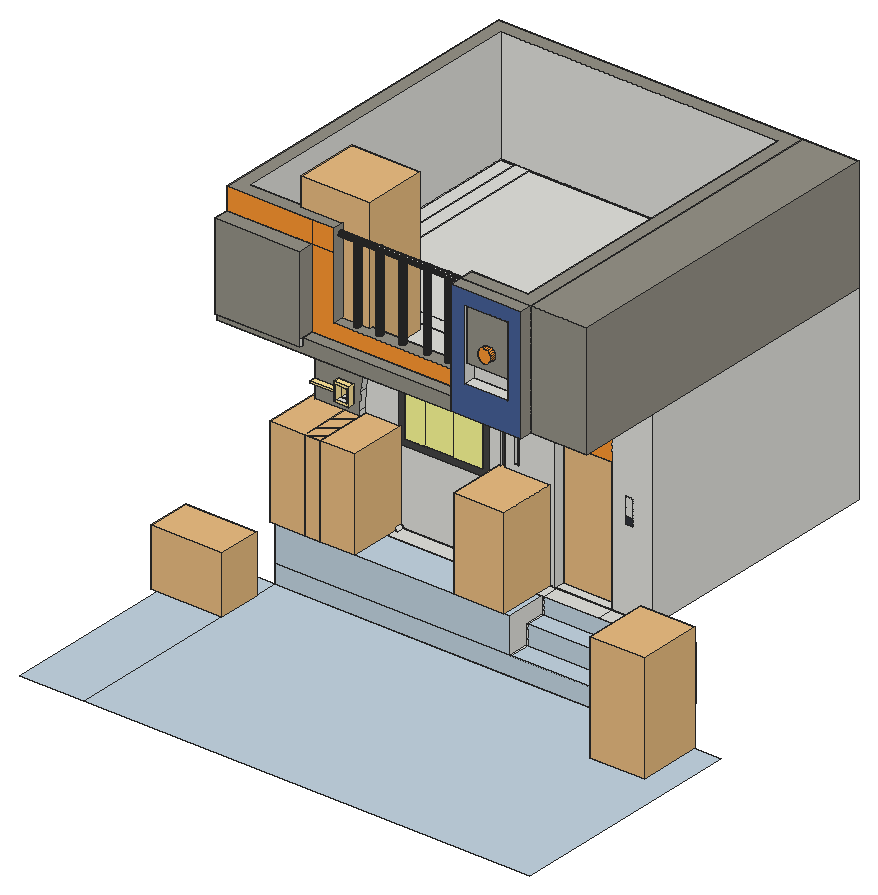
# SketchUp Ruby script. Lengths in inches.
U = 1.inch
M = Sketchup.active_model
def pt(a) = Geom::Point3d.new(a.map { |v| v * U })
def face(e, loops, mat)
  f = e.add_face(loops[0].map { |a| pt(a) })
  loops[1..].each { |l| e.add_face(l.map { |a| pt(a) }).erase! }
  f.material = f.back_material = mat if mat
  f
end
# faces: each face lists its corners as indices into pts; further lists are holes
def faces(e, pts, list, mat = nil) = list.each { |f| face(e, (f[0].is_a?(Array) ? f : [f]).map { |l| l.map { |i| pts[i] } }, mat) }
# xy, xz, yz: faces in a plane at the given z, y or x. An outline is a flat list of corners, or four numbers for a rectangle; further outlines are holes
def ring(l) = l.size == 4 ? [[l[0], l[1]], [l[2], l[1]], [l[2], l[3]], [l[0], l[3]]] : l.each_slice(2).to_a
def flat(e, list, mat, &to3) = list.each { |f| face(e, (f[0].is_a?(Array) ? f : [f]).map { |l| ring(l).map { |u, v| to3.(u, v) } }, mat) }
def xy(e, z, list, mat = nil) = flat(e, list, mat) { |x, y| [x, y, z] }
def xz(e, y, list, mat = nil) = flat(e, list, mat) { |x, z| [x, y, z] }
def yz(e, x, list, mat = nil) = flat(e, list, mat) { |y, z| [x, y, z] }
def lines(e, pts, list) = list.each { |a, b| e.add_line(pt(pts[a]), pt(pts[b])) }
# prism: a flat outline (further loops are holes) pulled along v
def prism(e, loops, v, mat = nil)
  f = face(e, loops, mat); d = Geom::Vector3d.new(v.map { |x| x * U })
  f.pushpull(f.normal.samedirection?(d) ? d.length : -d.length)
end
def box(e, o, s, mat = nil) = prism(e, [[o, [o[0] + s[0], o[1], o[2]], [o[0] + s[0], o[1] + s[1], o[2]], [o[0], o[1] + s[1], o[2]]]], [0, 0, s[2]], mat)
def at(x, y, z, deg = 0) = Geom::Transformation.translation(pt([x, y, z])) * Geom::Transformation.rotation(ORIGIN, Z_AXIS, deg.degrees)
def axes(o, x, y, z) = Geom::Transformation.new([*x, 0, *y, 0, *z, 0, *pt(o).to_a, 1])
def part(name) = M.definitions.add(name)
# library, detail: a bought-in or finely detailed component or shape, given as its bounding box
def library(name, o, s) = part(name).tap { |d| box(d.entities, o, s) }
def detail(e, o, s) = box(e.add_group.entities, o, s)
def put(e, d, t, mat = nil) = e.add_instance(d, t).tap { |i| i.material = mat if mat }
def group(e, t, mat = nil) = e.add_group.tap { |g| g.transformation = t; g.material = mat if mat }.entities
root = M.entities
M.materials.add("[Color C04]").color = [255, 153, 50]
M.materials.add("[Color D02]").color = [255, 229, 153]
M.materials.add("[Color E02]").color = [255, 255, 153]
M.materials.add("[Formica Blue]").color = [71, 97, 152]
M.materials.add("[Formica Graystone]").color = [149, 146, 135]
M.materials.add("[Formica Laminate Dark]").color = [50, 53, 60]
M.materials.add("[Granite Dark Gray]").color = [69, 68, 68]
M.materials.add("[Terrazzo Light Blue]").color = [196, 214, 227]
c1 = library("Decorative Plant",[-0.35,-0.24,0],[4.14,4.48,6.875])
c2 = library("blómastandur (1)",[6.48,-34.53,1.97],[34.7,40.11,68.37])
c3 = library("plantas+internas",[0,0,0],[44.91,27.47,36.11])
c4 = library("Door",[183.55,487.57,0],[5.16,42.5,84])
xy(root,-34.375,[[40.65,150.875,189.96,186.6875],[189.96,150.875,277.77,186.6875]])
xy(root,-34.375,[[0,0,40.65,150.875],[40.65,0,322.27,150.875]],"[Terrazzo Light Blue]")
xy(root,-22.29,[[40.65,150.875,189.02,163.875],[189.02,150.875,189.96,163.875]])
xy(root,-22.29,[[189.96,150.875,277.77,163.875]],"[Terrazzo Light Blue]")
xy(root,-10.2,[[40.65,163.875,189.02,176.1875],[189.02,163.875,189.96,176.1875]])
xy(root,-10.2,[[189.96,163.875,277.77,176.1875]],"[Terrazzo Light Blue]")
xy(root,0,[[40.65,176.1875,189.96,176.1875,189.96,186.6875,93.13,186.6875,93.13,182.375,40.65,182.375],[189.96,176.1875,225.02,186.6875],[225.02,176.1875,250.96,186.6875],[250.96,176.1875,277.77,186.6875],[40.65,182.375,93.13,186.6875],
  [40.65,186.6875,40.65,349.1875,250.96,349.1875,250.96,186.6875,225.02,186.6875,225.02,195.6875,241.96,195.6875,241.96,340.1875,49.65,340.1875,49.65,195.6875,189.02,195.6875,189.02,186.6875],[189.02,186.6875,225.02,195.6875],[49.65,195.6875,241.96,340.1875]])
xy(root,0,[[40.65,150.5625,189.02,176.1875]],"[Terrazzo Light Blue]")
xy(root,29.77,[[55.61,182.375,65.29,186.6875]])
xy(root,29.77,[[55.61,178.4375,65.29,182.375]],"[Color D02]")
xy(root,31.08,[[56.93,178.4375,63.97,182.375],[56.93,182.375,63.97,186.6875]],"[Color D02]")
xy(root,34.99,[[40.65,182.375,55.61,186.6875]])
xy(root,34.99,[[40.65,178.4375,55.61,182.375]],"[Color D02]")
xy(root,36.67,[[40.65,182.375,55.61,186.6875]])
xy(root,36.67,[[40.65,178.4375,55.61,182.375]],"[Color D02]")
xy(root,39.6875,[[154.5625,186.6875,157,188]])
xy(root,39.9375,[[56.93,178.4375,63.97,182.375],[56.93,182.375,63.97,186.6875]],"[Color D02]")
xy(root,41.25,[[55.61,182.375,65.29,186.6875]])
xy(root,41.25,[[55.61,178.4375,65.29,182.375]],"[Color D02]")
xy(root,51.2,[[93.97,186.6875,143.27,195.6875]])
xy(root,61.125,[[163.3,186.6875,166.05,188.1875]])
xy(root,62.33,[[55.61,182.375,65.29,186.6875]])
xy(root,62.33,[[55.61,178.4375,65.29,182.375]],"[Color D02]")
xy(root,63.64,[[56.93,178.4375,63.97,182.375],[56.93,182.375,63.97,186.6875]])
xy(root,67.54,[[40.65,182.375,55.61,186.6875],[40.65,186.6875,55.61,186.9375]])
xy(root,67.54,[[40.65,178.4375,55.61,182.375]],"[Color D02]")
xy(root,68.76,[[40.65,182.375,55.61,186.6875],[40.65,186.6875,55.61,186.9375]])
xy(root,68.76,[[40.65,178.4375,55.61,182.375]],"[Color D02]")
xy(root,72.5,[[56.93,178.4375,63.97,182.375],[56.93,182.375,63.97,186.6875]],"[Color D02]")
xy(root,73.8125,[[55.61,182.375,65.29,186.6875]])
xy(root,73.8125,[[55.61,178.4375,65.29,182.375]],"[Color D02]")
xy(root,84,[[189.02,186.6875,225.02,195.6875]])
xy(root,87.9375,[[171.8,186.6875,174.67,187.875]])
xy(root,89.08,[[55.61,182.375,65.29,186.6875]])
xy(root,89.08,[[55.61,178.4375,65.29,182.375]],"[Color D02]")
xy(root,90.39,[[56.93,178.4375,63.97,182.375],[56.93,182.375,63.97,186.6875]])
xy(root,93.49,[[93.97,186.6875,143.27,195.6875,143.27,186.6875],[93.97,186.6875,93.97,195.6875,143.27,195.6875]])
xy(root,94.2,[[40.65,182.375,55.61,185.875],[40.65,185.875,55.61,186.6875]])
xy(root,94.2,[[40.65,178.4375,55.61,182.375]],"[Color D02]")
xy(root,95.88,[[40.65,182.375,55.61,185.875],[40.65,185.875,55.61,186.6875]])
xy(root,95.88,[[40.65,178.4375,55.61,182.375]],"[Color D02]")
xy(root,99.25,[[56.93,178.4375,63.97,182.375],[56.93,182.375,63.97,186.6875]],"[Color D02]")
xy(root,100.5625,[[55.61,182.375,65.29,186.6875]])
xy(root,100.5625,[[55.61,178.4375,65.29,182.375]],"[Color D02]")
xy(root,120,[[40.65,182.375,93.13,186.6875],[[40.65,186.6875,154.5625,186.6875,154.5625,188,157,188,157,186.6875,163.3,186.6875,163.3,188.1875,166.05,188.1875,166.05,186.6875,171.8,186.6875,171.8,187.875,174.67,187.875,174.67,186.6875,250.96,186.6875,250.96,349.1875,40.65,349.1875],[49.65,195.6875,241.96,340.1875]]])
xz(root,150.875,[[40.65,-34.375,277.77,-22.29]],"[Terrazzo Light Blue]")
xz(root,163.875,[[40.65,-22.29,189.02,-10.2],[189.02,-22.29,189.96,-10.2]])
xz(root,163.875,[[189.96,-22.29,277.77,-10.2]],"[Terrazzo Light Blue]")
xz(root,176.1875,[[40.65,-10.2,189.02,0],[189.02,-10.2,189.96,0]])
xz(root,176.1875,[[189.96,-10.2,277.77,0]],"[Terrazzo Light Blue]")
xz(root,178.4375,[[[55.61,29.77,65.29,41.25],[56.93,31.08,63.97,39.9375]],[40.65,34.99,55.61,36.67],[[55.61,62.33,65.29,73.8125],[56.93,63.64,63.97,72.5]],[40.65,67.54,55.61,68.76],[[55.61,89.08,65.29,100.5625],[56.93,90.39,63.97,99.25]],
  [40.65,94.2,55.61,95.88]],"[Color D02]")
xz(root,182.375,[[[55.61,29.77,65.29,41.25],[56.93,31.08,63.97,39.9375]],[40.65,34.99,55.61,36.67],[[55.61,62.33,65.29,73.8125],[56.93,63.64,63.97,72.5]],[40.65,67.54,55.61,68.76],[[55.61,89.08,65.29,100.5625],[56.93,90.39,63.97,99.25]],
  [40.65,94.2,55.61,95.88]])
xz(root,182.375,[[40.65,0,93.13,0,85.93,8.4,79.86,17.65,75.04,27.61,71.53,38.1,69.41,48.96,68.7,60,69.41,71.04,71.53,81.9,75.04,92.39,79.86,102.35,85.93,111.6,93.13,120,40.65,120,40.65,95.88,55.61,95.88,55.61,100.5625,65.29,100.5625,65.29,89.08,55.61,89.08,55.61,94.2,40.65,94.2,40.65,68.76,55.61,68.76,55.61,73.8125,65.29,73.8125,65.29,62.33,55.61,62.33,55.61,67.54,40.65,67.54,40.65,36.67,55.61,36.67,55.61,41.25,65.29,41.25,65.29,29.77,55.61,29.77,55.61,34.99,40.65,34.99]],"[Formica Graystone]")
xz(root,185.875,[[40.65,94.2,55.61,95.88]])
xz(root,186.6875,[[40.65,-34.375,189.96,-22.29],[189.96,-34.375,277.77,-22.29],[40.65,-22.29,189.96,-10.2],[189.96,-22.29,277.77,-10.2],[40.65,-10.2,189.96,0],
  [189.96,-10.2,277.77,0],[40.65,0,40.65,34.99,55.61,34.99,55.61,29.77,65.29,29.77,65.29,41.25,55.61,41.25,55.61,36.67,40.65,36.67,40.65,67.54,55.61,67.54,55.61,62.33,65.29,62.33,65.29,73.8125,55.61,73.8125,55.61,68.76,40.65,68.76,40.65,94.2,55.61,94.2,55.61,89.08,65.29,89.08,65.29,100.5625,55.61,100.5625,55.61,95.88,40.65,95.88,40.65,120,93.13,120,85.93,111.6,79.86,102.35,75.04,92.39,71.53,81.9,69.41,71.04,68.7,60,69.41,48.96,71.53,38.1,75.04,27.61,79.86,17.65,85.93,8.4,93.13,0],[[93.13,0,189.02,0,189.02,120,174.67,120,174.67,87.9375,171.8,87.9375,171.8,120,166.05,120,166.05,61.125,163.3,61.125,163.3,120,157,120,157,39.6875,154.5625,39.6875,154.5625,120,93.13,120,85.93,111.6,79.86,102.35,75.04,92.39,71.53,81.9,69.41,71.04,68.7,60,69.41,48.96,71.53,38.1,75.04,27.61,79.86,17.65,85.93,8.4],[89.43,46.66,147.81,98.03]],[[225.02,0,250.96,120],[233.58,51.97,238.4,67.6]],[[55.61,29.77,65.29,41.25],[56.93,31.08,63.97,39.9375]],
  [56.93,31.08,63.97,39.9375],[40.65,34.99,55.61,36.67],[233.58,56.22,238.4,67.6],[[55.61,62.33,65.29,73.8125],[56.93,63.64,63.97,72.5]],[56.93,63.64,63.97,72.5],
  [40.65,67.54,55.61,68.76],[[55.61,89.08,65.29,100.5625],[56.93,90.39,63.97,99.25]],[56.93,90.39,63.97,99.25],[40.65,94.2,55.61,95.88]])
xz(root,186.6875,[[189.02,84,225.02,120]],"[Color C04]")
xz(root,186.6875,[[93.97,51.2,106.85,93.49],[106.85,51.2,125.06,93.49],[125.06,51.2,143.27,93.49]],"[Color E02]")
xz(root,186.6875,[[233.58,51.97,238.4,56.22]],"[Formica Laminate Dark]")
xz(root,186.6875,[[[89.43,46.66,147.81,98.03],[93.97,51.2,143.27,93.49]]],"[Granite Dark Gray]")
xz(root,186.9375,[[40.65,67.54,55.61,68.76]])
xz(root,187.875,[[171.8,87.9375,174.67,120]],"[Granite Dark Gray]")
xz(root,188,[[154.5625,39.6875,157,120]],"[Granite Dark Gray]")
xz(root,188.1875,[[163.3,61.125,166.05,120]],"[Granite Dark Gray]")
xz(root,195.6875,[[[49.65,0,49.65,120,241.96,120,241.96,0,225.02,0,225.02,84,189.02,84,189.02,0],[93.97,51.2,143.27,93.49]]])
xz(root,340.1875,[[49.65,0,241.96,120]])
xz(root,349.1875,[[40.65,0,250.96,120]])
yz(root,40.65,[[150.875,-34.375,150.875,-22.29,163.875,-22.29,163.875,-10.2,176.1875,-10.2,176.1875,0,182.375,0,182.375,-32.39,186.6875,-34.375],[186.6875,-34.375,182.375,-32.39,182.375,0,186.6875,0],[150.875,-22.29,150.5625,0,176.1875,0,176.1875,-10.2,163.875,-10.2,163.875,-22.29],[182.375,0,186.6875,34.99],[186.6875,0,186.6875,67.54,186.9375,67.54,186.9375,68.76,186.6875,68.76,186.6875,120,349.1875,120,349.1875,0],
  [178.4375,34.99,182.375,36.67],[182.375,34.99,186.6875,36.67],[182.375,36.67,186.6875,67.54],[178.4375,67.54,182.375,68.76],[182.375,67.54,186.6875,68.76],
  [186.6875,67.54,186.9375,68.76],[182.375,68.76,186.6875,94.2],[182.375,94.2,185.875,95.88],[185.875,94.2,186.6875,95.88],[182.375,95.88,186.6875,120]])
yz(root,40.65,[[178.4375,94.2,182.375,95.88]],"[Color D02]")
yz(root,49.65,[[195.6875,0,340.1875,120]])
yz(root,55.61,[[178.4375,29.77,182.375,34.99],[182.375,29.77,186.6875,34.99],[178.4375,34.99,182.375,36.67],[182.375,34.99,186.6875,36.67],[178.4375,36.67,182.375,41.25],
  [182.375,36.67,186.6875,41.25],[182.375,62.33,186.6875,67.54],[178.4375,67.54,182.375,68.76],[182.375,67.54,186.6875,68.76],[186.6875,67.54,186.9375,68.76],
  [182.375,68.76,186.6875,73.8125],[182.375,89.08,186.6875,94.2],[178.4375,94.2,182.375,95.88],[182.375,94.2,185.875,95.88],[185.875,94.2,186.6875,95.88],
  [182.375,95.88,186.6875,100.5625]])
yz(root,55.61,[[178.4375,62.33,182.375,67.54],[178.4375,68.76,182.375,73.8125],[178.4375,89.08,182.375,94.2],[178.4375,95.88,182.375,100.5625]],"[Color D02]")
yz(root,56.93,[[178.4375,31.08,182.375,39.9375],[182.375,31.08,186.6875,39.9375],[178.4375,63.64,182.375,72.5],[182.375,63.64,186.6875,72.5],[178.4375,90.39,182.375,99.25],
  [182.375,90.39,186.6875,99.25]],"[Color D02]")
yz(root,63.97,[[178.4375,31.08,182.375,39.9375],[182.375,31.08,186.6875,39.9375],[178.4375,63.64,182.375,72.5],[182.375,63.64,186.6875,72.5],[178.4375,90.39,182.375,99.25],
  [182.375,90.39,186.6875,99.25]],"[Color D02]")
yz(root,65.29,[[178.4375,29.77,182.375,41.25],[182.375,29.77,186.6875,41.25],[182.375,62.33,186.6875,73.8125],[182.375,89.08,186.6875,100.5625]])
yz(root,65.29,[[178.4375,62.33,182.375,73.8125],[178.4375,89.08,182.375,100.5625]],"[Color D02]")
yz(root,93.97,[[186.6875,51.2,195.6875,93.49]])
yz(root,143.27,[[186.6875,51.2,195.6875,93.49]])
yz(root,154.5625,[[186.6875,39.6875,188,120]])
yz(root,157,[[186.6875,39.6875,188,120]])
yz(root,163.3,[[186.6875,61.125,188.1875,120]])
yz(root,166.05,[[186.6875,61.125,188.1875,120]])
yz(root,171.8,[[186.6875,87.9375,187.875,120]])
yz(root,174.67,[[186.6875,87.9375,187.875,120]])
yz(root,189.02,[[150.875,-22.29,163.875,-22.29,163.875,-10.2,176.1875,-10.2,176.1875,0,150.5625,0],[186.6875,0,195.6875,84]])
yz(root,225.02,[[186.6875,0,195.6875,84]])
yz(root,241.96,[[195.6875,0,340.1875,120]])
yz(root,250.96,[[186.6875,0,349.1875,120]])
yz(root,277.77,[[150.875,-34.375,186.6875,-22.29],[163.875,-22.29,186.6875,-10.2],[176.1875,-10.2,186.6875,0]])
p = [[189.02,150.875,-22.29],[189.02,150.5625,0],[40.65,150.5625,0],[40.65,150.875,-22.29],[93.13,186.6875,0],[85.93,186.6875,8.4],
  [85.93,182.375,8.4],[93.13,182.375,0],[79.86,186.6875,17.65],[79.86,182.375,17.65],[75.04,186.6875,27.61],[75.04,182.375,27.61],
  [71.53,186.6875,38.1],[71.53,182.375,38.1],[69.41,186.6875,48.96],[69.41,182.375,48.96],[68.7,186.6875,60],[68.7,182.375,60],
  [69.41,186.6875,71.04],[69.41,182.375,71.04],[71.53,186.6875,81.9],[71.53,182.375,81.9],[75.04,186.6875,92.39],[75.04,182.375,92.39],
  [79.86,186.6875,102.35],[79.86,182.375,102.35],[85.93,186.6875,111.6],[85.93,182.375,111.6],[93.13,186.6875,120],[93.13,182.375,120]]
faces(root,p,[[0,1,2,3]],"[Terrazzo Light Blue]")
faces(root,p,[[4,5,6,7],[5,8,9,6],[8,10,11,9],[10,12,13,11],[12,14,15,13],[14,16,17,15],[16,18,19,17],[18,20,21,19],
  [20,22,23,21],[22,24,25,23],[24,26,27,25],[26,28,29,27]])
put(root,c1,axes([156.35,152.67,0],[7.66714,0,0],[0,8.94221,0],[0,0,8.3288]))
put(root,c1,axes([40.45,152.67,0],[7.66714,0,0],[0,8.94221,0],[0,0,8.3288]))
put(root,c1,axes([62.23,152.67,0],[7.66714,0,0],[0,8.94221,0],[0,0,8.3288]))
put(root,c2,at(266.57,143.39,-34.375))
put(root,c3,at(-4.26,108.69,-34.375))
put(root,c4,axes([-232.24,106.66,84.19],[0,0.47177,0],[0.864,0,0],[0,0,-1.00226]))
put(root,c1,axes([68.35,143.46,119.75],[10.4273,0,0],[0,8.94221,0],[0,0,13.02624]))
g1 = group(root,at(23.15,125,119.75))
xy(g1,0,[[[0,9.5625,192.3125,224.19],[8.55,18.11,183.76,215.64]],[8.55,18.11,183.76,215.64]])
xy(g1,0.25,[[0,1.75,67.8,9.5625],[67.8,1.75,147.8125,9.5625],[147.8125,1.75,192.3125,9.5625],[0,9.5625,0,224.19,192.3125,224.19,192.3125,9.5625,147.8125,9.5625,147.8125,18.11,183.76,18.11,183.76,215.64,8.55,215.64,8.55,18.11,67.8,18.11,67.8,9.5625],[67.8,9.5625,147.8125,18.11]])
xy(g1,0.25,[[192.3125,9.5625,227.8125,224.19]],"[Formica Graystone]")
xy(g1,4.45,[[0,0,54.0625,1.75],[0,1.75,54.0625,9.5625]])
xy(g1,8.87,[[54.0625,1.75,147.8125,9.5625]],"[Formica Graystone]")
xy(g1,18.76,[[156.43,1.75,183.69,9.5625],[78.79,12.74,78.32,12.8,77.88,12.98,77.51,13.27,77.22,13.64,77.04,14.08,76.98,14.55,77.04,15.02,77.22,15.45,77.51,15.83,77.88,16.12,78.32,16.3,78.79,16.36,79.26,16.3,79.7,16.12,80.07,15.83,80.36,15.45,80.54,15.02,80.6,14.55,80.54,14.08,80.36,13.64,80.07,13.27,79.7,12.98,79.26,12.8],[92.79,12.74,92.32,12.8,91.88,12.98,91.51,13.27,91.22,13.64,91.04,14.08,90.98,14.55,91.04,15.02,91.22,15.45,91.51,15.83,91.88,16.12,92.32,16.3,92.79,16.36,93.26,16.3,93.7,16.12,94.07,15.83,94.36,15.45,94.54,15.02,94.6,14.55,94.54,14.08,94.36,13.64,94.07,13.27,93.7,12.98,93.26,12.8],[107.23,12.74,106.76,12.8,106.32,12.98,105.95,13.27,105.66,13.64,105.48,14.08,105.42,14.55,105.48,15.02,105.66,15.45,105.95,15.83,106.32,16.12,106.76,16.3,107.23,16.36,107.7,16.3,108.13,16.12,108.51,15.83,108.8,15.45,108.98,15.02,109.04,14.55,108.98,14.08,108.8,13.64,108.51,13.27,108.13,12.98,107.7,12.8],[122.79,12.74,122.32,12.8,121.88,12.98,121.51,13.27,121.22,13.64,121.04,14.08,120.98,14.55,121.04,15.02,121.22,15.45,121.51,15.83,121.88,16.12,122.32,16.3,122.79,16.36,123.26,16.3,123.7,16.12,124.07,15.83,124.36,15.45,124.54,15.02,124.6,14.55,124.54,14.08,124.36,13.64,124.07,13.27,123.7,12.98,123.26,12.8],
  [136.04,12.74,135.57,12.8,135.13,12.98,134.76,13.27,134.47,13.64,134.29,14.08,134.23,14.55,134.29,15.02,134.47,15.45,134.76,15.83,135.13,16.12,135.57,16.3,136.04,16.36,136.51,16.3,136.95,16.12,137.32,15.83,137.61,15.45,137.79,15.02,137.85,14.55,137.79,14.08,137.61,13.64,137.32,13.27,136.95,12.98,136.51,12.8]])
xy(g1,18.76,[[[67.8,9.5625,147.8125,18.11],[107.23,12.74,106.76,12.8,106.32,12.98,105.95,13.27,105.66,13.64,105.48,14.08,105.42,14.55,105.48,15.02,105.66,15.45,105.95,15.83,106.32,16.12,106.76,16.3,107.23,16.36,107.7,16.3,108.13,16.12,108.51,15.83,108.8,15.45,108.98,15.02,109.04,14.55,108.98,14.08,108.8,13.64,108.51,13.27,108.13,12.98,107.7,12.8],[122.79,12.74,122.32,12.8,121.88,12.98,121.51,13.27,121.22,13.64,121.04,14.08,120.98,14.55,121.04,15.02,121.22,15.45,121.51,15.83,121.88,16.12,122.32,16.3,122.79,16.36,123.26,16.3,123.7,16.12,124.07,15.83,124.36,15.45,124.54,15.02,124.6,14.55,124.54,14.08,124.36,13.64,124.07,13.27,123.7,12.98,123.26,12.8],[78.79,12.74,78.32,12.8,77.88,12.98,77.51,13.27,77.22,13.64,77.04,14.08,76.98,14.55,77.04,15.02,77.22,15.45,77.51,15.83,77.88,16.12,78.32,16.3,78.79,16.36,79.26,16.3,79.7,16.12,80.07,15.83,80.36,15.45,80.54,15.02,80.6,14.55,80.54,14.08,80.36,13.64,80.07,13.27,79.7,12.98,79.26,12.8],[92.79,12.74,92.32,12.8,91.88,12.98,91.51,13.27,91.22,13.64,91.04,14.08,90.98,14.55,91.04,15.02,91.22,15.45,91.51,15.83,91.88,16.12,92.32,16.3,92.79,16.36,93.26,16.3,93.7,16.12,94.07,15.83,94.36,15.45,94.54,15.02,94.6,14.55,94.54,14.08,94.36,13.64,94.07,13.27,93.7,12.98,93.26,12.8],[136.04,12.74,135.57,12.8,135.13,12.98,134.76,13.27,134.47,13.64,134.29,14.08,134.23,14.55,134.29,15.02,134.47,15.45,134.76,15.83,135.13,16.12,135.57,16.3,136.04,16.36,136.51,16.3,136.95,16.12,137.32,15.83,137.61,15.45,137.79,15.02,137.85,14.55,137.79,14.08,137.61,13.64,137.32,13.27,136.95,12.98,136.51,12.8]]],"[Formica Graystone]")
xy(g1,29.58,[[156.43,3.75,183.69,9.5625]])
xy(g1,58.51,[[0,0,54.0625,9.5625]],"[Formica Graystone]")
xy(g1,63.63,[[156.43,1.75,183.69,3.75],[156.43,3.75,183.69,9.5625]])
xy(g1,67.43,[[78.79,12.74,79.26,12.8,79.7,12.98,80.07,13.27,80.36,13.64,80.54,14.08,80.6,14.55,80.54,15.02,80.36,15.45,80.28,15.5625,77.31,15.5625,77.22,15.45,77.04,15.02,76.98,14.55,77.04,14.08,77.22,13.64,77.51,13.27,77.88,12.98,78.32,12.8],[107.23,12.74,107.7,12.8,108.13,12.98,108.51,13.27,108.8,13.64,108.98,14.08,109.04,14.55,108.98,15.02,108.8,15.45,108.71,15.5625,105.74,15.5625,105.66,15.45,105.48,15.02,105.42,14.55,105.48,14.08,105.66,13.64,105.95,13.27,106.32,12.98,106.76,12.8],[77.31,15.5625,80.28,15.5625,80.07,15.83,79.7,16.12,79.26,16.3,78.79,16.36,78.32,16.3,77.88,16.12,77.51,15.83],[105.74,15.5625,108.71,15.5625,108.51,15.83,108.13,16.12,107.7,16.3,107.23,16.36,106.76,16.3,106.32,16.12,105.95,15.83]])
xy(g1,68.27,[[92.79,12.74,93.26,12.8,93.7,12.98,94.07,13.27,94.36,13.64,94.54,14.08,94.6,14.55,94.54,15.02,94.36,15.45,94.28,15.5625,91.31,15.5625,91.22,15.45,91.04,15.02,90.98,14.55,91.04,14.08,91.22,13.64,91.51,13.27,91.88,12.98,92.32,12.8],[122.79,12.74,123.26,12.8,123.7,12.98,124.07,13.27,124.36,13.64,124.54,14.08,124.6,14.55,124.54,15.02,124.36,15.45,124.28,15.5625,121.31,15.5625,121.22,15.45,121.04,15.02,120.98,14.55,121.04,14.08,121.22,13.64,121.51,13.27,121.88,12.98,122.32,12.8],[91.31,15.5625,94.28,15.5625,94.07,15.83,93.7,16.12,93.26,16.3,92.79,16.36,92.32,16.3,91.88,16.12,91.51,15.83],[121.31,15.5625,124.28,15.5625,124.07,15.83,123.7,16.12,123.26,16.3,122.79,16.36,122.32,16.3,121.88,16.12,121.51,15.83]])
xy(g1,68.66,[[136.04,12.74,136.51,12.8,136.95,12.98,137.32,13.27,137.61,13.64,137.79,14.08,137.85,14.55,137.79,15.02,137.63,15.4,134.45,15.4,134.29,15.02,134.23,14.55,134.29,14.08,134.47,13.64,134.76,13.27,135.13,12.98,135.57,12.8],[134.45,15.4,137.63,15.4,137.61,15.45,137.32,15.83,136.95,16.12,136.51,16.3,136.04,16.36,135.57,16.3,135.13,16.12,134.76,15.83,134.47,15.45]])
xy(g1,72.25,[[147.8125,1.75,192.3125,9.5625],[0,9.5625,67.8,9.5625,67.8,18.11,8.55,18.11,8.55,215.64,183.76,215.64,183.76,18.11,147.8125,18.11,147.8125,9.5625,192.3125,9.5625,192.3125,224.19,0,224.19],[192.3125,9.5625,227.8125,224.19]],"[Formica Graystone]")
xz(g1,0,[[0,4.45,54.0625,58.51]],"[Formica Graystone]")
xz(g1,0.375,[[170.15,35.6,171.25,35.75,172.27,36.17,173.15,36.85,173.83,37.73,174.25,38.75,174.4,39.85,174.25,40.95,173.83,41.98,173.15,42.86,172.27,43.53,171.25,43.96,170.15,44.1,169.05,43.96,168.02,43.53,167.14,42.86,166.47,41.98,166.04,40.95,165.9,39.85,166.04,38.75,166.47,37.73,167.14,36.85,168.02,36.17,169.05,35.75]],"[Color C04]")
xz(g1,1.75,[[[147.8125,0.25,192.3125,72.25],[156.43,18.76,183.69,63.63]]],"[Formica Blue]")
xz(g1,1.75,[[0,0.25,147.8125,0.25,147.8125,8.87,54.0625,8.87,54.0625,4.45,0,4.45]],"[Formica Graystone]")
xz(g1,3.75,[[170.15,35.6,169.05,35.75,168.02,36.17,167.14,36.85,166.47,37.73,166.04,38.75,165.9,39.85,166.04,40.95,166.47,41.98,167.14,42.86,168.02,43.53,169.05,43.96,170.15,44.1,171.25,43.96,172.27,43.53,173.15,42.86,173.83,41.98,174.25,40.95,174.4,39.85,174.25,38.75,173.83,37.73,173.15,36.85,172.27,36.17,171.25,35.75]])
xz(g1,3.75,[[[156.43,29.58,183.69,63.63],[170.15,35.6,169.05,35.75,168.02,36.17,167.14,36.85,166.47,37.73,166.04,38.75,165.9,39.85,166.04,40.95,166.47,41.98,167.14,42.86,168.02,43.53,169.05,43.96,170.15,44.1,171.25,43.96,172.27,43.53,173.15,42.86,173.83,41.98,174.25,40.95,174.4,39.85,174.25,38.75,173.83,37.73,173.15,36.85,172.27,36.17,171.25,35.75]]],"[Formica Graystone]")
xz(g1,9.5625,[[0,0,192.3125,0.25],[0,0.25,0,4.45,54.0625,4.45,54.0625,8.87,183.69,8.87,183.69,63.63,156.43,63.63,156.43,18.76,147.8125,18.76,147.8125,72.25,192.3125,72.25,192.3125,0.25],[0,4.45,54.0625,58.51],[147.8125,8.87,156.43,18.76],[156.43,8.87,183.69,18.76],
  [156.43,18.76,183.69,29.58],[156.43,29.58,183.69,63.63]])
xz(g1,9.5625,[[54.0625,8.87,147.8125,8.87,147.8125,18.76,67.8,18.76,67.8,58.51,54.0625,58.51],[0,58.51,54.0625,72.25],[54.0625,58.51,67.8,72.25]],"[Color C04]")
xz(g1,9.5625,[[192.3125,0.25,227.8125,72.25]],"[Formica Graystone]")
xz(g1,18.11,[[8.55,0,67.8,0.25],[67.8,0,147.8125,0.25],[147.8125,0,183.76,0.25],[8.55,0.25,67.8,72.25],[67.8,0.25,147.8125,18.76],
  [147.8125,0.25,183.76,72.25]])
xz(g1,215.64,[[8.55,0,183.76,0.25],[8.55,0.25,183.76,72.25]])
xz(g1,224.19,[[0,0,192.3125,0.25]])
xz(g1,224.19,[[0,0.25,192.3125,72.25],[192.3125,0.25,227.8125,72.25]],"[Formica Graystone]")
yz(g1,0,[[9.5625,0,224.19,0.25]])
yz(g1,0,[[1.75,0.25,9.5625,4.45],[9.5625,0.25,224.19,72.25],[0,4.45,9.5625,58.51]],"[Formica Graystone]")
yz(g1,8.55,[[18.11,0,215.64,0.25],[18.11,0.25,215.64,72.25]])
yz(g1,54.0625,[[0,4.45,1.75,8.87],[1.75,4.45,9.5625,8.87]])
yz(g1,54.0625,[[0,8.87,9.5625,58.51]],"[Formica Graystone]")
yz(g1,67.8,[[13.99,66.23,13.57,66.28,13.18,66.45,12.85,66.7,12.59,67.04,12.42,67.43,12.37,67.85,12.42,68.27,12.59,68.66,12.85,69,13.18,69.26,13.57,69.42,13.99,69.48,14.42,69.42,14.81,69.26,15.14,69,15.4,68.66,15.5625,68.27,15.62,67.85,15.5625,67.43,15.4,67.04,15.14,66.7,14.81,66.45,14.42,66.28]])
yz(g1,67.8,[[[9.5625,18.76,18.11,72.25],[13.99,66.23,13.57,66.28,13.18,66.45,12.85,66.7,12.59,67.04,12.42,67.43,12.37,67.85,12.42,68.27,12.59,68.66,12.85,69,13.18,69.26,13.57,69.42,13.99,69.48,14.42,69.42,14.81,69.26,15.14,69,15.4,68.66,15.5625,68.27,15.62,67.85,15.5625,67.43,15.4,67.04,15.14,66.7,14.81,66.45,14.42,66.28]]],"[Formica Graystone]")
yz(g1,147.8125,[[18.11,0,9.5625,0.25,18.11,0.25],[1.75,0.25,1.75,8.87,9.5625,8.87,9.5625,18.76,18.11,18.76,18.11,0.25]])
yz(g1,147.8125,[[1.75,8.87,9.5625,18.76],[1.75,18.76,9.5625,72.25],[[9.5625,18.76,18.11,72.25],[13.99,66.23,14.42,66.28,14.81,66.45,15.14,66.7,15.4,67.04,15.5625,67.43,15.62,67.85,15.5625,68.27,15.4,68.66,15.14,69,14.81,69.26,14.42,69.42,13.99,69.48,13.57,69.42,13.18,69.26,12.85,69,12.59,68.66,12.42,68.27,12.37,67.85,12.42,67.43,12.59,67.04,12.85,66.7,13.18,66.45,13.57,66.28]]],"[Formica Graystone]")
yz(g1,156.43,[[1.75,18.76,9.5625,18.76,9.5625,29.58,3.75,29.58,3.75,63.63,1.75,63.63],[3.75,29.58,9.5625,63.63]])
yz(g1,183.69,[[1.75,18.76,1.75,63.63,3.75,63.63,3.75,29.58,9.5625,29.58,9.5625,18.76],[3.75,29.58,9.5625,63.63]])
yz(g1,183.76,[[18.11,0,215.64,0.25],[18.11,0.25,215.64,72.25]])
yz(g1,192.3125,[[9.5625,0,224.19,0.25]])
yz(g1,192.3125,[[1.75,0.25,9.5625,72.25],[9.5625,0.25,224.19,72.25]],"[Formica Graystone]")
yz(g1,227.8125,[[9.5625,0.25,224.19,72.25]],"[Formica Graystone]")
p = [[78.32,12.8,18.76],[78.79,12.74,18.76],[78.79,12.74,67.43],[78.32,12.8,67.43],[79.26,12.8,18.76],[79.26,12.8,67.43],
  [92.32,12.8,18.76],[92.79,12.74,18.76],[92.79,12.74,68.27],[92.32,12.8,68.27],[93.26,12.8,18.76],[93.26,12.8,68.27],
  [106.76,12.8,18.76],[107.23,12.74,18.76],[107.23,12.74,67.43],[106.76,12.8,67.43],[107.7,12.8,18.76],[107.7,12.8,67.43],
  [122.32,12.8,18.76],[122.79,12.74,18.76],[122.79,12.74,68.27],[122.32,12.8,68.27],[123.26,12.8,18.76],[123.26,12.8,68.27],
  [135.57,12.8,18.76],[136.04,12.74,18.76],[136.04,12.74,68.66],[135.57,12.8,68.66],[136.51,12.8,18.76],[136.51,12.8,68.66],
  [77.88,12.98,18.76],[77.88,12.98,67.43],[79.7,12.98,18.76],[79.7,12.98,67.43],[91.88,12.98,18.76],[91.88,12.98,68.27],
  [93.7,12.98,18.76],[93.7,12.98,68.27],[106.32,12.98,18.76],[106.32,12.98,67.43],[108.13,12.98,18.76],[108.13,12.98,67.43],
  [121.88,12.98,18.76],[121.88,12.98,68.27],[123.7,12.98,18.76],[123.7,12.98,68.27],[135.13,12.98,18.76],[135.13,12.98,68.66],
  [136.95,12.98,18.76],[136.95,12.98,68.66],[77.51,13.27,18.76],[77.51,13.27,67.43],[80.07,13.27,18.76],[80.07,13.27,67.43],
  [91.51,13.27,18.76],[91.51,13.27,68.27],[94.07,13.27,18.76],[94.07,13.27,68.27],[105.95,13.27,18.76],[105.95,13.27,67.43],
  [108.51,13.27,18.76],[108.51,13.27,67.43],[121.51,13.27,18.76],[121.51,13.27,68.27],[124.07,13.27,18.76],[124.07,13.27,68.27],
  [134.76,13.27,18.76],[134.76,13.27,68.66],[137.32,13.27,18.76],[137.32,13.27,68.66],[77.22,13.64,18.76],[77.22,13.64,67.43],
  [80.36,13.64,18.76],[80.36,13.64,67.43],[91.22,13.64,18.76],[91.22,13.64,68.27],[94.36,13.64,18.76],[94.36,13.64,68.27],
  [105.66,13.64,18.76],[105.66,13.64,67.43],[108.8,13.64,18.76],[108.8,13.64,67.43],[121.22,13.64,18.76],[121.22,13.64,68.27],
  [124.36,13.64,18.76],[124.36,13.64,68.27],[134.47,13.64,18.76],[134.47,13.64,68.66],[137.61,13.64,18.76],[137.61,13.64,68.66],
  [77.04,14.08,18.76],[77.04,14.08,67.43],[80.54,14.08,18.76],[80.54,14.08,67.43],[91.04,14.08,18.76],[91.04,14.08,68.27],
  [94.54,14.08,18.76],[94.54,14.08,68.27],[105.48,14.08,18.76],[105.48,14.08,67.43],[108.98,14.08,18.76],[108.98,14.08,67.43],
  [121.04,14.08,18.76],[121.04,14.08,68.27],[124.54,14.08,18.76],[124.54,14.08,68.27],[134.29,14.08,18.76],[134.29,14.08,68.66],
  [137.79,14.08,18.76],[137.79,14.08,68.66],[76.98,14.55,18.76],[76.98,14.55,67.43],[80.6,14.55,18.76],[80.6,14.55,67.43],
  [90.98,14.55,18.76],[90.98,14.55,68.27],[94.6,14.55,18.76],[94.6,14.55,68.27],[105.42,14.55,18.76],[105.42,14.55,67.43],
  [109.04,14.55,18.76],[109.04,14.55,67.43],[120.98,14.55,18.76],[120.98,14.55,68.27],[124.6,14.55,18.76],[124.6,14.55,68.27],
  [134.23,14.55,18.76],[134.23,14.55,68.66],[137.85,14.55,18.76],[137.85,14.55,68.66],[77.04,15.02,18.76],[77.04,15.02,67.43],
  [80.54,15.02,18.76],[80.54,15.02,67.43],[91.04,15.02,18.76],[91.04,15.02,68.27],[94.54,15.02,18.76],[94.54,15.02,68.27],
  [105.48,15.02,18.76],[105.48,15.02,67.43],[108.98,15.02,18.76],[108.98,15.02,67.43],[121.04,15.02,18.76],[121.04,15.02,68.27],
  [124.54,15.02,18.76],[124.54,15.02,68.27],[134.29,15.02,18.76],[134.29,15.02,68.66],[137.79,15.02,18.76],[137.79,15.02,68.66],
  [77.22,15.45,18.76],[77.22,15.45,67.43],[80.36,15.45,18.76],[80.36,15.45,67.43],[91.22,15.45,18.76],[91.22,15.45,68.27],
  [94.36,15.45,18.76],[94.36,15.45,68.27],[105.66,15.45,18.76],[105.66,15.45,67.43],[108.8,15.45,18.76],[108.8,15.45,67.43],
  [121.22,15.45,18.76],[121.22,15.45,68.27],[124.36,15.45,18.76],[124.36,15.45,68.27],[134.47,15.45,18.76],[134.45,15.4,68.66],
  [134.47,15.45,68.66],[137.61,15.45,18.76],[137.61,15.45,68.66],[137.63,15.4,68.66],[77.51,15.83,18.76],[77.31,15.5625,67.43],
  [77.51,15.83,67.43],[80.07,15.83,18.76],[80.07,15.83,67.43],[80.28,15.5625,67.43],[91.51,15.83,18.76],[91.31,15.5625,68.27],
  [91.51,15.83,68.27],[94.07,15.83,18.76],[94.07,15.83,68.27],[94.28,15.5625,68.27],[105.95,15.83,18.76],[105.74,15.5625,67.43],
  [105.95,15.83,67.43],[108.51,15.83,18.76],[108.51,15.83,67.43],[108.71,15.5625,67.43],[121.51,15.83,18.76],[121.31,15.5625,68.27],
  [121.51,15.83,68.27],[124.07,15.83,18.76],[124.07,15.83,68.27],[124.28,15.5625,68.27],[134.76,15.83,18.76],[134.76,15.83,68.66],
  [137.32,15.83,18.76],[137.32,15.83,68.66],[77.88,16.12,18.76],[77.88,16.12,67.43],[79.7,16.12,18.76],[79.7,16.12,67.43],
  [91.88,16.12,18.76],[91.88,16.12,68.27],[93.7,16.12,18.76],[93.7,16.12,68.27],[106.32,16.12,18.76],[106.32,16.12,67.43],
  [108.13,16.12,18.76],[108.13,16.12,67.43],[121.88,16.12,18.76],[121.88,16.12,68.27],[123.7,16.12,18.76],[123.7,16.12,68.27],
  [135.13,16.12,18.76],[135.13,16.12,68.66],[136.95,16.12,18.76],[136.95,16.12,68.66],[78.32,16.3,18.76],[78.32,16.3,67.43],
  [79.26,16.3,18.76],[79.26,16.3,67.43],[92.32,16.3,18.76],[92.32,16.3,68.27],[93.26,16.3,18.76],[93.26,16.3,68.27],
  [106.76,16.3,18.76],[106.76,16.3,67.43],[107.7,16.3,18.76],[107.7,16.3,67.43],[122.32,16.3,18.76],[122.32,16.3,68.27],
  [123.26,16.3,18.76],[123.26,16.3,68.27],[135.57,16.3,18.76],[135.57,16.3,68.66],[136.51,16.3,18.76],[136.51,16.3,68.66],
  [78.79,16.36,18.76],[78.79,16.36,67.43],[92.79,16.36,18.76],[92.79,16.36,68.27],[107.23,16.36,18.76],[107.23,16.36,67.43],
  [122.79,16.36,18.76],[122.79,16.36,68.27],[136.04,16.36,18.76],[136.04,16.36,68.66],[169.05,3.75,35.75],[170.15,3.75,35.6],
  [170.15,0.375,35.6],[169.05,0.375,35.75],[171.25,3.75,35.75],[171.25,0.375,35.75],[168.02,3.75,36.17],[168.02,0.375,36.17],
  [172.27,3.75,36.17],[172.27,0.375,36.17],[167.14,3.75,36.85],[167.14,0.375,36.85],[173.15,3.75,36.85],[173.15,0.375,36.85],
  [166.47,3.75,37.73],[166.47,0.375,37.73],[173.83,3.75,37.73],[173.83,0.375,37.73],[166.04,3.75,38.75],[166.04,0.375,38.75],
  [174.25,3.75,38.75],[174.25,0.375,38.75],[165.9,3.75,39.85],[165.9,0.375,39.85],[174.4,3.75,39.85],[174.4,0.375,39.85],
  [166.04,3.75,40.95],[166.04,0.375,40.95],[174.25,3.75,40.95],[174.25,0.375,40.95],[166.47,3.75,41.98],[166.47,0.375,41.98],
  [173.83,3.75,41.98],[173.83,0.375,41.98],[167.14,3.75,42.86],[167.14,0.375,42.86],[173.15,3.75,42.86],[173.15,0.375,42.86],
  [168.02,3.75,43.53],[168.02,0.375,43.53],[172.27,3.75,43.53],[172.27,0.375,43.53],[169.05,3.75,43.96],[169.05,0.375,43.96],
  [171.25,3.75,43.96],[171.25,0.375,43.96],[170.15,3.75,44.1],[170.15,0.375,44.1],[67.8,13.57,66.28],[67.8,13.99,66.23],
  [147.8125,13.99,66.23],[147.8125,13.57,66.28],[67.8,14.42,66.28],[147.8125,14.42,66.28],[67.8,13.18,66.45],[147.8125,13.18,66.45],
  [67.8,14.81,66.45],[147.8125,14.81,66.45],[67.8,12.85,66.7],[147.8125,12.85,66.7],[67.8,15.14,66.7],[147.8125,15.14,66.7],
  [67.8,12.59,67.04],[147.8125,12.59,67.04],[67.8,15.4,67.04],[147.8125,15.4,67.04],[67.8,12.42,67.43],[147.8125,12.42,67.43],
  [67.8,15.5625,67.43],[147.8125,15.5625,67.43],[67.8,12.37,67.85],[147.8125,12.37,67.85],[67.8,15.62,67.85],[147.8125,15.62,67.85],
  [67.8,12.42,68.27],[147.8125,12.42,68.27],[67.8,15.5625,68.27],[147.8125,15.5625,68.27],[67.8,12.59,68.66],[147.8125,12.59,68.66],
  [67.8,15.4,68.66],[147.8125,15.4,68.66],[67.8,12.85,69],[147.8125,12.85,69],[67.8,15.14,69],[147.8125,15.14,69],
  [67.8,13.18,69.26],[147.8125,13.18,69.26],[67.8,14.81,69.26],[147.8125,14.81,69.26],[67.8,13.57,69.42],[147.8125,13.57,69.42],
  [67.8,14.42,69.42],[147.8125,14.42,69.42],[67.8,13.99,69.48],[147.8125,13.99,69.48],[183.69,9.5625,8.87],[183.69,1.75,8.87],
  [156.43,9.5625,8.87],[156.43,1.75,8.87]]
faces(g1,p,[[0,1,2,3],[1,4,5,2],[6,7,8,9],[7,10,11,8],[12,13,14,15],[13,16,17,14],[18,19,20,21],[19,22,23,20],
  [24,25,26,27],[25,28,29,26],[30,0,3,31],[4,32,33,5],[34,6,9,35],[10,36,37,11],[38,12,15,39],[16,40,41,17],
  [42,18,21,43],[22,44,45,23],[46,24,27,47],[28,48,49,29],[50,30,31,51],[32,52,53,33],[54,34,35,55],[36,56,57,37],
  [58,38,39,59],[40,60,61,41],[62,42,43,63],[44,64,65,45],[66,46,47,67],[48,68,69,49],[70,50,51,71],[52,72,73,53],
  [74,54,55,75],[56,76,77,57],[78,58,59,79],[60,80,81,61],[82,62,63,83],[64,84,85,65],[86,66,67,87],[68,88,89,69],
  [90,70,71,91],[72,92,93,73],[94,74,75,95],[76,96,97,77],[98,78,79,99],[80,100,101,81],[102,82,83,103],[84,104,105,85],
  [106,86,87,107],[88,108,109,89],[110,90,91,111],[92,112,113,93],[114,94,95,115],[96,116,117,97],[118,98,99,119],[100,120,121,101],
  [122,102,103,123],[104,124,125,105],[126,106,107,127],[108,128,129,109],[130,110,111,131],[112,132,133,113],[134,114,115,135],[116,136,137,117],
  [138,118,119,139],[120,140,141,121],[142,122,123,143],[124,144,145,125],[146,126,127,147],[128,148,149,129],[150,130,131,151],[132,152,153,133],
  [154,134,135,155],[136,156,157,137],[158,138,139,159],[140,160,161,141],[162,142,143,163],[144,164,165,145],[166,146,147,167,168],[148,169,170,171,149],
  [172,150,151,173,174],[152,175,176,177,153],[178,154,155,179,180],[156,181,182,183,157],[184,158,159,185,186],[160,187,188,189,161],[190,162,163,191,192],[164,193,194,195,165],
  [196,166,168,197],[169,198,199,170],[200,172,174,201],[175,202,203,176],[204,178,180,205],[181,206,207,182],[208,184,186,209],[187,210,211,188],
  [212,190,192,213],[193,214,215,194],[216,196,197,217],[198,218,219,199],[220,200,201,221],[202,222,223,203],[224,204,205,225],[206,226,227,207],
  [228,208,209,229],[210,230,231,211],[232,212,213,233],[214,234,235,215],[236,216,217,237],[218,238,239,219],[240,220,221,241],[222,240,241,223],
  [242,224,225,243],[226,242,243,227],[244,228,229,245],[230,244,245,231],[246,232,233,247],[234,246,247,235],[248,236,237,249],[238,248,249,239],
  [298,299,300,301],[299,302,303,300],[304,298,301,305],[302,306,307,303],[308,304,305,309],[306,310,311,307],[312,308,309,313],[310,314,315,311],
  [316,312,313,317],[314,318,173,177,185,189,319,315],[320,316,317,321],[318,322,323,319,189,185,177,173],[324,320,321,325],[322,326,179,183,191,195,327,323],[328,324,325,329],[326,330,167,171,331,327,195,191,183,179],
  [332,328,329,333],[330,334,335,331,171,167],[336,332,333,337],[334,338,339,335],[340,336,337,341],[338,342,343,339],[344,340,341,345],[342,344,345,343]])
faces(g1,p,[[250,251,252,253],[251,254,255,252],[256,250,253,257],[254,258,259,255],[260,256,257,261],[258,262,263,259],[264,260,261,265],[262,266,267,263],
  [268,264,265,269],[266,270,271,267],[272,268,269,273],[270,274,275,271],[276,272,273,277],[274,278,279,275],[280,276,277,281],[278,282,283,279],
  [284,280,281,285],[282,286,287,283],[288,284,285,289],[286,290,291,287],[292,288,289,293],[290,294,295,291],[296,292,293,297],[294,296,297,295]],"[Color C04]")
lines(g1,p,[[346,347],[348,349]])
